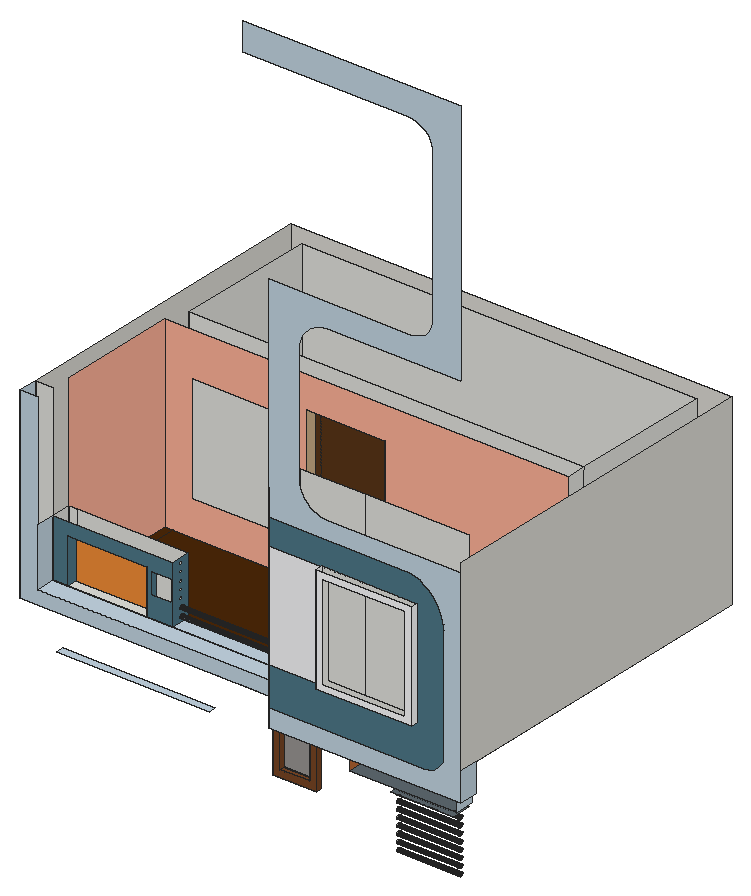
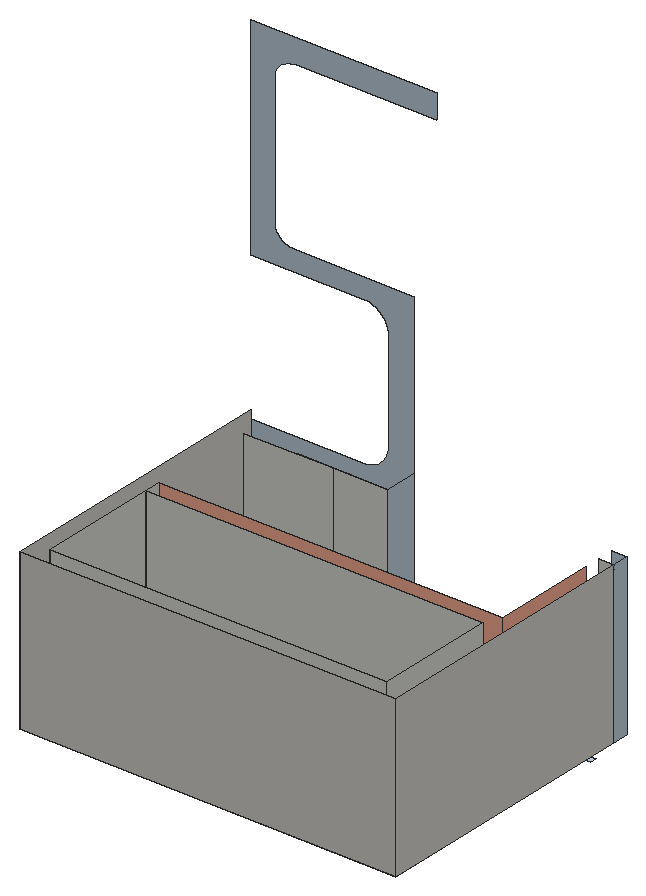
# SketchUp Ruby script. Lengths in inches.
U = 1.inch
M = Sketchup.active_model
def pt(a) = Geom::Point3d.new(a.map { |v| v * U })
def face(e, loops, mat)
  f = e.add_face(loops[0].map { |a| pt(a) })
  loops[1..].each { |l| e.add_face(l.map { |a| pt(a) }).erase! }
  f.material = f.back_material = mat if mat
  f
end
# faces: each face lists its corners as indices into pts; further lists are holes
def faces(e, pts, list, mat = nil) = list.each { |f| face(e, (f[0].is_a?(Array) ? f : [f]).map { |l| l.map { |i| pts[i] } }, mat) }
# xy, xz, yz: faces in a plane at the given z, y or x. An outline is a flat list of corners, or four numbers for a rectangle; further outlines are holes
def ring(l) = l.size == 4 ? [[l[0], l[1]], [l[2], l[1]], [l[2], l[3]], [l[0], l[3]]] : l.each_slice(2).to_a
def flat(e, list, mat, &to3) = list.each { |f| face(e, (f[0].is_a?(Array) ? f : [f]).map { |l| ring(l).map { |u, v| to3.(u, v) } }, mat) }
def xy(e, z, list, mat = nil) = flat(e, list, mat) { |x, y| [x, y, z] }
def xz(e, y, list, mat = nil) = flat(e, list, mat) { |x, z| [x, y, z] }
def yz(e, x, list, mat = nil) = flat(e, list, mat) { |y, z| [x, y, z] }
def lines(e, pts, list) = list.each { |a, b| e.add_line(pt(pts[a]), pt(pts[b])) }
# prism: a flat outline (further loops are holes) pulled along v
def prism(e, loops, v, mat = nil)
  f = face(e, loops, mat); d = Geom::Vector3d.new(v.map { |x| x * U })
  f.pushpull(f.normal.samedirection?(d) ? d.length : -d.length)
end
def box(e, o, s, mat = nil) = prism(e, [[o, [o[0] + s[0], o[1], o[2]], [o[0] + s[0], o[1] + s[1], o[2]], [o[0], o[1] + s[1], o[2]]]], [0, 0, s[2]], mat)
def at(x, y, z, deg = 0) = Geom::Transformation.translation(pt([x, y, z])) * Geom::Transformation.rotation(ORIGIN, Z_AXIS, deg.degrees)
def axes(o, x, y, z) = Geom::Transformation.new([*x, 0, *y, 0, *z, 0, *pt(o).to_a, 1])
def part(name) = M.definitions.add(name)
# library, detail: a bought-in or finely detailed component or shape, given as its bounding box
def library(name, o, s) = part(name).tap { |d| box(d.entities, o, s) }
def detail(e, o, s) = box(e.add_group.entities, o, s)
def put(e, d, t, mat = nil) = e.add_instance(d, t).tap { |i| i.material = mat if mat }
def group(e, t, mat = nil) = e.add_group.tap { |g| g.transformation = t; g.material = mat if mat }.entities
root = M.entities
M.materials.add("[0035_Tan]").color = [210, 180, 140]
M.materials.add("[0096_SkyBlue]").color = [79, 120, 137]
M.materials.add("[Blinds Vertical Pattern]").color = [247, 247, 249]
M.materials.add("[Cladding Siding Tan]").color = [242, 141, 55]
M.materials.add("[Color B02]").color = [255, 178, 153]
M.materials.add("[Concrete Aggregate Smoke]").color = [154, 150, 148]
M.materials.add("[Formica Laminate Dark]").color = [50, 53, 60]
M.materials.add("[Formica Speckled Grey]").color = [94, 105, 111]
M.materials.add("[Leather Red Brown]").color = [76, 40, 8]
M.materials.add("[Quartz Light Grey]").color = [251, 251, 252]
M.materials.add("[Terrazzo Light Blue]").color = [196, 214, 227]
M.materials.add("[Terrazzo Tile Light]").color = [219, 217, 210]
M.materials.add("[Wood Cherry Original]").color = [188, 106, 52]
M.materials.add("[Wood Floor Parquet]").color = [89, 54, 24]
M.materials.add("[Wood Veneer 01]").color = [120, 70, 37]
xy(root,101.78,[[212.44,171.81,240.69,175.06]],"[Wood Veneer 01]")
xy(root,106.21,[[216.87,171.81,236.26,175.06]],"[Wood Veneer 01]")
xy(root,116.03,[[285.76,175.06,326.14,187.5]],"[Formica Speckled Grey]")
xy(root,119,[[259.37,175.06,326.14,187.5],[326.14,175.06,328.05,187.5]],"[Formica Speckled Grey]")
xy(root,129.14,[[79.41,164.37,177.78,169]],"[Terrazzo Light Blue]")
xy(root,129.79,[[216.87,171.81,236.26,175.06]],"[Wood Veneer 01]")
xy(root,134.22,[[212.44,171.81,240.69,175.06]],"[Wood Veneer 01]")
xy(root,134.25,[[217.34,162.87,340.49,175.06]],"[Terrazzo Light Blue]")
xy(root,142.25,[[259.37,175.06,328.05,187.5]])
xy(root,152.8125,[[57.16,162.87,73.72,169],[73.72,162.87,210.68,169],[210.68,162.87,217.34,175.06],[57.16,169,73.72,175.06],[73.72,169,210.68,175.06],
  [73.72,175.06,217.34,187.5],[217.34,175.06,328.05,187.5],[73.72,277.89,328.05,368.29]])
xy(root,152.8125,[[159.93,265.26,209.68,271.64]],"[0035_Tan]")
xy(root,152.8125,[[73.72,265.26,73.72,277.89,328.05,277.89,328.05,265.26,209.68,265.26,209.68,271.64,159.93,271.64,159.93,265.26]],"[Formica Speckled Grey]")
xy(root,152.8125,[[57.16,175.06,57.16,380.73,340.49,380.73,340.49,175.06,328.05,175.06,328.05,368.29,73.72,368.29,73.72,265.26,68.53,265.26,68.53,187.5,73.72,187.5,73.72,175.06],[68.53,187.5,73.72,265.26],[73.72,187.5,328.05,265.26]],"[Leather Red Brown]")
xy(root,161.75,[[68.53,175.06,68.53,187.5,145.53,187.5,145.53,175.06,129.11,175.06,129.11,181.62,77.92,181.62,77.92,175.06],[77.92,175.06,129.11,181.62]])
xy(root,161.75,[[68.53,162.87,217.34,175.06],[145.53,175.06,217.34,187.5]],"[Terrazzo Light Blue]")
xy(root,170.49,[[250.99,158.43,312.37,162.87]],"[Quartz Light Grey]")
xz(root,158.43,[[[250.99,170.49,312.37,239.3],[254.96,174.45,308.4,235.33]]],"[Quartz Light Grey]")
xz(root,162.87,[[[250.99,170.49,312.37,239.3],[254.96,174.45,308.4,235.33]]])
xz(root,162.87,[[217.34,145.51,317.89,145.51,319.24,145.59,320.59,145.84,321.89,146.24,323.15,146.8,324.35,147.51,325.47,148.35,326.49,149.33,327.41,150.42,328.21,151.62,328.89,152.9,329.4375,154.26,329.84,155.67,329.84,227.94,329.62,231.55,328.97,235.1,327.91,238.53,326.4375,241.77,324.6,244.78,322.41,247.5,319.91,249.88,317.15,251.89,314.17,253.49,311.03,254.66,307.78,255.36,304.46,255.6,217.34,255.6,217.34,239.3,312.37,239.3,312.37,170.49,217.34,170.49]],"[0096_SkyBlue]")
xz(root,162.87,[[217.34,170.49,250.99,239.3]],"[Blinds Vertical Pattern]")
xz(root,162.87,[[217.34,134.25,340.49,134.25,340.49,266.71,254.82,266.71,252.4375,266.86,250.1,267.33,247.84,268.09,245.71,269.15,243.72,270.47,241.93,272.04,240.36,273.84,239.04,275.82,237.98,277.95,237.22,280.21,236.75,282.55,236.6,284.93,236.6,358.97,236.75,361.36,237.22,363.71,237.99,365.98,239.05,368.13,240.38,370.125,241.97,371.93,243.77,373.51,245.76,374.84,247.91,375.9,250.18,376.67,252.54,377.14,254.93,377.3,340.49,377.3,340.49,536.0625,200.4,536.0625,200.4,518.04,306.125,518.04,308.3,517.92,310.4375,517.55,312.5,516.9375,314.45,516.1,316.26,515.05,317.9,513.8,319.34,512.375,320.55,510.8,321.51,509.1,322.21,507.31,322.64,505.45,322.78,503.56,322.78,405.53,322.65,403.87,322.28,402.24,321.67,400.66,320.82,399.17,319.76,397.79,318.5,396.54,317.06,395.44,315.47,394.52,313.75,393.78,311.9375,393.25,310.0625,392.92,308.15,392.8125,217.34,392.8125,217.34,255.6,304.46,255.6,307.78,255.36,311.03,254.66,314.17,253.49,317.15,251.89,319.91,249.88,322.41,247.5,324.6,244.78,326.4375,241.77,327.91,238.53,328.97,235.1,329.62,231.55,329.84,227.94,329.84,155.67,329.4375,154.26,328.89,152.9,328.21,151.62,327.41,150.42,326.49,149.33,325.47,148.35,324.35,147.51,323.15,146.8,321.89,146.24,320.59,145.84,319.24,145.59,317.89,145.51,217.34,145.51],[57.16,152.8125,217.34,152.8125,217.34,161.75,68.53,161.75,68.53,272.8125,57.16,272.8125]],"[Terrazzo Light Blue]")
xz(root,171.81,[[[212.44,101.78,240.69,134.22],[216.87,106.21,236.26,129.79]]],"[Wood Veneer 01]")
xz(root,175.06,[[[212.44,101.78,240.69,134.22],[216.87,106.21,236.26,129.79]],[217.34,134.25,259.37,134.25,259.37,142.25,328.05,142.25,328.05,152.8125,217.34,152.8125],[259.37,134.25,328.05,142.25],[328.05,134.25,340.49,142.25],[328.05,142.25,340.49,152.8125],
  [57.16,152.8125,57.16,272.8125,68.53,272.8125,68.53,161.75,217.34,161.75,217.34,152.8125]])
xz(root,175.06,[[[68.53,161.75,77.92,161.75,77.92,190.75,129.11,190.75,129.11,161.75,145.53,161.75,145.53,199,68.53,199],[131.3,175.61,144.73,189.05]]],"[0096_SkyBlue]")
xz(root,175.06,[[216.87,106.21,236.26,129.79]],"[Concrete Aggregate Smoke]")
xz(root,181.62,[[77.92,161.75,129.11,190.75]],"[Cladding Siding Tan]")
xz(root,187.5,[[68.53,152.8125,73.72,161.75],[73.72,152.8125,217.34,161.75],[217.34,152.8125,259.37,272.8125],[259.37,152.8125,326.14,272.8125],[68.53,161.75,73.72,199],
  [73.72,161.75,145.53,199]])
xz(root,265.26,[[[68.53,152.8125,159.93,152.8125,159.93,252.25,209.68,252.25,209.68,152.8125,328.05,152.8125,328.05,272.8125,68.53,272.8125],[85.49,175.17,140.61,244.54]]],"[Color B02]")
xz(root,271.64,[[[159.93,152.8125,209.68,252.25],[163.48,156.36,206.13,248.7]],[163.48,156.36,206.13,248.7]],"[Wood Floor Parquet]")
xz(root,277.89,[[73.72,152.8125,328.05,272.8125]])
xz(root,368.29,[[73.72,152.8125,328.05,272.8125]])
xz(root,380.73,[[57.16,152.8125,340.49,272.8125]],"[Terrazzo Tile Light]")
yz(root,57.16,[[162.87,152.8125,175.06,272.8125]],"[Terrazzo Light Blue]")
yz(root,57.16,[[175.06,152.8125,380.73,272.8125]],"[Terrazzo Tile Light]")
yz(root,68.53,[[175.06,161.75,187.5,199]])
yz(root,68.53,[[187.5,152.8125,265.26,272.8125]],"[Color B02]")
yz(root,68.53,[[162.87,161.75,175.06,199]],"[Terrazzo Light Blue]")
yz(root,73.72,[[277.89,152.8125,368.29,272.8125]])
yz(root,77.92,[[175.06,161.75,181.62,190.75]],"[0096_SkyBlue]")
yz(root,129.11,[[175.06,161.75,181.62,190.75]],"[0096_SkyBlue]")
yz(root,145.53,[[181.52,164.09,181.21,164.125,180.92,164.24,180.68,164.43,180.49,164.68,180.37,164.97,180.33,165.27,180.37,165.58,180.49,165.87,180.68,166.11,180.92,166.3,181.21,166.42,181.52,166.46,181.82,166.42,182.11,166.3,182.35,166.11,182.54,165.87,182.66,165.58,182.7,165.27,182.66,164.97,182.54,164.68,182.35,164.43,182.11,164.24,181.82,164.125],[181.52,169.34,181.21,169.375,180.92,169.49,180.68,169.68,180.49,169.93,180.37,170.22,180.33,170.52,180.37,170.83,180.49,171.12,180.68,171.36,180.92,171.55,181.21,171.67,181.52,171.71,181.82,171.67,182.11,171.55,182.35,171.36,182.54,171.12,182.66,170.83,182.7,170.52,182.66,170.22,182.54,169.93,182.35,169.68,182.11,169.49,181.82,169.375]])
yz(root,145.53,[[[175.06,161.75,187.5,199],[181.52,164.09,181.21,164.125,180.92,164.24,180.68,164.43,180.49,164.68,180.37,164.97,180.33,165.27,180.37,165.58,180.49,165.87,180.68,166.11,180.92,166.3,181.21,166.42,181.52,166.46,181.82,166.42,182.11,166.3,182.35,166.11,182.54,165.87,182.66,165.58,182.7,165.27,182.66,164.97,182.54,164.68,182.35,164.43,182.11,164.24,181.82,164.125],[181.52,189.77,181.21,189.8125,180.92,189.93,180.68,190.12,180.49,190.37,180.37,190.65,180.33,190.96,180.37,191.27,180.49,191.55,180.68,191.8,180.92,191.99,181.21,192.11,181.52,192.15,181.82,192.11,182.11,191.99,182.35,191.8,182.54,191.55,182.66,191.27,182.7,190.96,182.66,190.65,182.54,190.37,182.35,190.12,182.11,189.93,181.82,189.8125],[181.52,169.34,181.21,169.375,180.92,169.49,180.68,169.68,180.49,169.93,180.37,170.22,180.33,170.52,180.37,170.83,180.49,171.12,180.68,171.36,180.92,171.55,181.21,171.67,181.52,171.71,181.82,171.67,182.11,171.55,182.35,171.36,182.54,171.12,182.66,170.83,182.7,170.52,182.66,170.22,182.54,169.93,182.35,169.68,182.11,169.49,181.82,169.375],[181.52,184.52,181.21,184.5625,180.92,184.68,180.68,184.87,180.49,185.12,180.37,185.4,180.33,185.71,180.37,186.02,180.49,186.3,180.68,186.55,180.92,186.74,181.21,186.86,181.52,186.9,181.82,186.86,182.11,186.74,182.35,186.55,182.54,186.3,182.66,186.02,182.7,185.71,182.66,185.4,182.54,185.12,182.35,184.87,182.11,184.68,181.82,184.5625],[181.52,174.46,181.21,174.5,180.92,174.62,180.68,174.81,180.49,175.05,180.37,175.34,180.33,175.65,180.37,175.96,180.49,176.24,180.68,176.49,180.92,176.68,181.21,176.8,181.52,176.84,181.82,176.8,182.11,176.68,182.35,176.49,182.54,176.24,182.66,175.96,182.7,175.65,182.66,175.34,182.54,175.05,182.35,174.81,182.11,174.62,181.82,174.5],[181.52,179.59,181.21,179.625,180.92,179.74,180.68,179.93,180.49,180.18,180.37,180.47,180.33,180.77,180.37,181.08,180.49,181.37,180.68,181.61,180.92,181.8,181.21,181.92,181.52,181.96,181.82,181.92,182.11,181.8,182.35,181.61,182.54,181.37,182.66,181.08,182.7,180.77,182.66,180.47,182.54,180.18,182.35,179.93,182.11,179.74,181.82,179.625],[181.52,194.9,181.21,194.9375,180.92,195.06,180.68,195.25,180.49,195.49,180.37,195.78,180.33,196.09,180.37,196.39,180.49,196.68,180.68,196.93,180.92,197.11,181.21,197.23,181.52,197.27,181.82,197.23,182.11,197.11,182.35,196.93,182.54,196.68,182.66,196.39,182.7,196.09,182.66,195.78,182.54,195.49,182.35,195.25,182.11,195.06,181.82,194.9375]]],"[0096_SkyBlue]")
yz(root,159.93,[[265.26,152.8125,271.64,252.25]],"[0035_Tan]")
yz(root,209.68,[[265.26,152.8125,271.64,252.25]],"[0035_Tan]")
yz(root,212.44,[[171.81,101.78,175.06,134.22]],"[Wood Veneer 01]")
yz(root,216.87,[[171.81,106.21,175.06,129.79]],"[Wood Veneer 01]")
yz(root,217.34,[[162.87,134.25,175.06,152.8125],[162.87,152.8125,175.06,161.75],[175.06,152.8125,187.5,161.75]])
yz(root,217.34,[[[162.87,161.75,187.5,272.8125],[181.52,194.9,181.82,194.9375,182.11,195.06,182.35,195.25,182.54,195.49,182.66,195.78,182.7,196.09,182.66,196.39,182.54,196.68,182.35,196.93,182.11,197.11,181.82,197.23,181.52,197.27,181.21,197.23,180.92,197.11,180.68,196.93,180.49,196.68,180.37,196.39,180.33,196.09,180.37,195.78,180.49,195.49,180.68,195.25,180.92,195.06,181.21,194.9375],[181.52,164.09,181.82,164.125,182.11,164.24,182.35,164.43,182.54,164.68,182.66,164.97,182.7,165.27,182.66,165.58,182.54,165.87,182.35,166.11,182.11,166.3,181.82,166.42,181.52,166.46,181.21,166.42,180.92,166.3,180.68,166.11,180.49,165.87,180.37,165.58,180.33,165.27,180.37,164.97,180.49,164.68,180.68,164.43,180.92,164.24,181.21,164.125],[181.52,169.34,181.82,169.375,182.11,169.49,182.35,169.68,182.54,169.93,182.66,170.22,182.7,170.52,182.66,170.83,182.54,171.12,182.35,171.36,182.11,171.55,181.82,171.67,181.52,171.71,181.21,171.67,180.92,171.55,180.68,171.36,180.49,171.12,180.37,170.83,180.33,170.52,180.37,170.22,180.49,169.93,180.68,169.68,180.92,169.49,181.21,169.375],[181.52,174.46,181.82,174.5,182.11,174.62,182.35,174.81,182.54,175.05,182.66,175.34,182.7,175.65,182.66,175.96,182.54,176.24,182.35,176.49,182.11,176.68,181.82,176.8,181.52,176.84,181.21,176.8,180.92,176.68,180.68,176.49,180.49,176.24,180.37,175.96,180.33,175.65,180.37,175.34,180.49,175.05,180.68,174.81,180.92,174.62,181.21,174.5],[181.52,179.59,181.82,179.625,182.11,179.74,182.35,179.93,182.54,180.18,182.66,180.47,182.7,180.77,182.66,181.08,182.54,181.37,182.35,181.61,182.11,181.8,181.82,181.92,181.52,181.96,181.21,181.92,180.92,181.8,180.68,181.61,180.49,181.37,180.37,181.08,180.33,180.77,180.37,180.47,180.49,180.18,180.68,179.93,180.92,179.74,181.21,179.625],[181.52,184.52,181.82,184.5625,182.11,184.68,182.35,184.87,182.54,185.12,182.66,185.4,182.7,185.71,182.66,186.02,182.54,186.3,182.35,186.55,182.11,186.74,181.82,186.86,181.52,186.9,181.21,186.86,180.92,186.74,180.68,186.55,180.49,186.3,180.37,186.02,180.33,185.71,180.37,185.4,180.49,185.12,180.68,184.87,180.92,184.68,181.21,184.5625],[181.52,189.77,181.82,189.8125,182.11,189.93,182.35,190.12,182.54,190.37,182.66,190.65,182.7,190.96,182.66,191.27,182.54,191.55,182.35,191.8,182.11,191.99,181.82,192.11,181.52,192.15,181.21,192.11,180.92,191.99,180.68,191.8,180.49,191.55,180.37,191.27,180.33,190.96,180.37,190.65,180.49,190.37,180.68,190.12,180.92,189.93,181.21,189.8125]]],"[Terrazzo Light Blue]")
yz(root,236.26,[[171.81,106.21,175.06,129.79]],"[Wood Veneer 01]")
yz(root,240.69,[[171.81,101.78,175.06,134.22]],"[Wood Veneer 01]")
yz(root,250.99,[[158.43,170.49,162.87,239.3]],"[Quartz Light Grey]")
yz(root,259.37,[[175.06,119,187.5,142.25]],"[Wood Cherry Original]")
yz(root,285.76,[[181.25,78.9,180.96,78.94,180.6875,79.05,180.45,79.23,180.28,79.47,180.16,79.74,180.125,80.03,180.16,80.32,180.28,80.59,180.45,80.82,180.6875,81,180.96,81.12,181.25,81.15,181.54,81.12,181.8125,81,182.05,80.82,182.22,80.59,182.34,80.32,182.375,80.03,182.34,79.74,182.22,79.47,182.05,79.23,181.8125,79.05,181.54,78.94],[181.25,83.59,180.96,83.63,180.6875,83.74,180.45,83.92,180.28,84.15,180.16,84.42,180.125,84.72,180.16,85.01,180.28,85.28,180.45,85.51,180.6875,85.69,180.96,85.8,181.25,85.84,181.54,85.8,181.8125,85.69,182.05,85.51,182.22,85.28,182.34,85.01,182.375,84.72,182.34,84.42,182.22,84.15,182.05,83.92,181.8125,83.74,181.54,83.63],[181.25,88.28,180.96,88.32,180.6875,88.43,180.45,88.61,180.28,88.84,180.16,89.11,180.125,89.4,180.16,89.69,180.28,89.97,180.45,90.2,180.6875,90.38,180.96,90.49,181.25,90.53,181.54,90.49,181.8125,90.38,182.05,90.2,182.22,89.97,182.34,89.69,182.375,89.4,182.34,89.11,182.22,88.84,182.05,88.61,181.8125,88.43,181.54,88.32],[181.25,92.97,180.96,93,180.6875,93.12,180.45,93.3,180.28,93.53,180.16,93.8,180.125,94.09,180.16,94.38,180.28,94.65,180.45,94.89,180.6875,95.07,180.96,95.18,181.25,95.22,181.54,95.18,181.8125,95.07,182.05,94.89,182.22,94.65,182.34,94.38,182.375,94.09,182.34,93.8,182.22,93.53,182.05,93.3,181.8125,93.12,181.54,93],[181.25,97.65,180.96,97.69,180.6875,97.8,180.45,97.98,180.28,98.22,180.16,98.49,180.125,98.78,180.16,99.07,180.28,99.34,180.45,99.57,180.6875,99.75,180.96,99.87,181.25,99.9,181.54,99.87,181.8125,99.75,182.05,99.57,182.22,99.34,182.34,99.07,182.375,98.78,182.34,98.49,182.22,98.22,182.05,97.98,181.8125,97.8,181.54,97.69],
  [181.25,102.34,180.96,102.38,180.6875,102.49,180.45,102.67,180.28,102.9,180.16,103.17,180.125,103.47,180.16,103.76,180.28,104.03,180.45,104.26,180.6875,104.44,180.96,104.55,181.25,104.59,181.54,104.55,181.8125,104.44,182.05,104.26,182.22,104.03,182.34,103.76,182.375,103.47,182.34,103.17,182.22,102.9,182.05,102.67,181.8125,102.49,181.54,102.38],[181.25,107.03,180.96,107.07,180.6875,107.18,180.45,107.36,180.28,107.59,180.16,107.86,180.125,108.15,180.16,108.44,180.28,108.72,180.45,108.95,180.6875,109.13,180.96,109.24,181.25,109.28,181.54,109.24,181.8125,109.13,182.05,108.95,182.22,108.72,182.34,108.44,182.375,108.15,182.34,107.86,182.22,107.59,182.05,107.36,181.8125,107.18,181.54,107.07],[181.25,111.72,180.96,111.75,180.6875,111.87,180.45,112.05,180.28,112.28,180.16,112.55,180.125,112.84,180.16,113.13,180.28,113.4,180.45,113.64,180.6875,113.82,180.96,113.93,181.25,113.97,181.54,113.93,181.8125,113.82,182.05,113.64,182.22,113.4,182.34,113.13,182.375,112.84,182.34,112.55,182.22,112.28,182.05,112.05,181.8125,111.87,181.54,111.75]])
yz(root,312.37,[[158.43,170.49,162.87,239.3]],"[Quartz Light Grey]")
yz(root,328.05,[[175.06,142.25,187.5,152.8125],[265.26,152.8125,277.89,272.8125],[277.89,152.8125,368.29,272.8125]])
yz(root,328.05,[[175.06,119,187.5,142.25]],"[Terrazzo Light Blue]")
yz(root,340.49,[[162.87,134.25,175.06,152.8125]],"[Terrazzo Light Blue]")
yz(root,340.49,[[162.87,152.8125,380.73,272.8125]],"[Terrazzo Tile Light]")
p = [[285.76,180.6875,79.05],[285.76,180.96,78.94],[326.14,180.96,78.94],[326.14,180.6875,79.05],[285.76,181.25,78.9],[326.14,181.25,78.9],
  [285.76,181.54,78.94],[326.14,181.54,78.94],[285.76,181.8125,79.05],[326.14,181.8125,79.05],[285.76,180.45,79.23],[326.14,180.45,79.23],
  [285.76,182.05,79.23],[326.14,182.05,79.23],[285.76,180.28,79.47],[326.14,180.28,79.47],[285.76,182.22,79.47],[326.14,182.22,79.47],
  [285.76,180.16,79.74],[326.14,180.16,79.74],[285.76,182.34,79.74],[326.14,182.34,79.74],[285.76,180.125,80.03],[326.14,180.125,80.03],
  [285.76,182.375,80.03],[326.14,182.375,80.03],[285.76,180.16,80.32],[326.14,180.16,80.32],[285.76,182.34,80.32],[326.14,182.34,80.32],
  [285.76,180.28,80.59],[326.14,180.28,80.59],[285.76,182.22,80.59],[326.14,182.22,80.59],[285.76,180.45,80.82],[326.14,180.45,80.82],
  [285.76,182.05,80.82],[326.14,182.05,80.82],[285.76,180.6875,81],[326.14,180.6875,81],[285.76,181.8125,81],[326.14,181.8125,81],
  [285.76,180.96,81.12],[326.14,180.96,81.12],[285.76,181.54,81.12],[326.14,181.54,81.12],[285.76,181.25,81.15],[326.14,181.25,81.15],
  [285.76,180.6875,83.74],[285.76,180.96,83.63],[326.14,180.96,83.63],[326.14,180.6875,83.74],[285.76,181.25,83.59],[326.14,181.25,83.59],
  [285.76,181.54,83.63],[326.14,181.54,83.63],[285.76,181.8125,83.74],[326.14,181.8125,83.74],[285.76,180.45,83.92],[326.14,180.45,83.92],
  [285.76,182.05,83.92],[326.14,182.05,83.92],[285.76,180.28,84.15],[326.14,180.28,84.15],[285.76,182.22,84.15],[326.14,182.22,84.15],
  [285.76,180.16,84.42],[326.14,180.16,84.42],[285.76,182.34,84.42],[326.14,182.34,84.42],[285.76,180.125,84.72],[326.14,180.125,84.72],
  [285.76,182.375,84.72],[326.14,182.375,84.72],[285.76,180.16,85.01],[326.14,180.16,85.01],[285.76,182.34,85.01],[326.14,182.34,85.01],
  [285.76,180.28,85.28],[326.14,180.28,85.28],[285.76,182.22,85.28],[326.14,182.22,85.28],[285.76,180.45,85.51],[326.14,180.45,85.51],
  [285.76,182.05,85.51],[326.14,182.05,85.51],[285.76,180.6875,85.69],[326.14,180.6875,85.69],[285.76,181.8125,85.69],[326.14,181.8125,85.69],
  [285.76,180.96,85.8],[326.14,180.96,85.8],[285.76,181.54,85.8],[326.14,181.54,85.8],[285.76,181.25,85.84],[326.14,181.25,85.84],
  [285.76,180.6875,88.43],[285.76,180.96,88.32],[326.14,180.96,88.32],[326.14,180.6875,88.43],[285.76,181.25,88.28],[326.14,181.25,88.28],
  [285.76,181.54,88.32],[326.14,181.54,88.32],[285.76,181.8125,88.43],[326.14,181.8125,88.43],[285.76,180.45,88.61],[326.14,180.45,88.61],
  [285.76,182.05,88.61],[326.14,182.05,88.61],[285.76,180.28,88.84],[326.14,180.28,88.84],[285.76,182.22,88.84],[326.14,182.22,88.84],
  [285.76,180.16,89.11],[326.14,180.16,89.11],[285.76,182.34,89.11],[326.14,182.34,89.11],[285.76,180.125,89.4],[326.14,180.125,89.4],
  [285.76,182.375,89.4],[326.14,182.375,89.4],[285.76,180.16,89.69],[326.14,180.16,89.69],[285.76,182.34,89.69],[326.14,182.34,89.69],
  [285.76,180.28,89.97],[326.14,180.28,89.97],[285.76,182.22,89.97],[326.14,182.22,89.97],[285.76,180.45,90.2],[326.14,180.45,90.2],
  [285.76,182.05,90.2],[326.14,182.05,90.2],[285.76,180.6875,90.38],[326.14,180.6875,90.38],[285.76,181.8125,90.38],[326.14,181.8125,90.38],
  [285.76,180.96,90.49],[326.14,180.96,90.49],[285.76,181.54,90.49],[326.14,181.54,90.49],[285.76,181.25,90.53],[326.14,181.25,90.53],
  [285.76,180.6875,93.12],[285.76,180.96,93],[326.14,180.96,93],[326.14,180.6875,93.12],[285.76,181.25,92.97],[326.14,181.25,92.97],
  [285.76,181.54,93],[326.14,181.54,93],[285.76,181.8125,93.12],[326.14,181.8125,93.12],[285.76,180.45,93.3],[326.14,180.45,93.3],
  [285.76,182.05,93.3],[326.14,182.05,93.3],[285.76,180.28,93.53],[326.14,180.28,93.53],[285.76,182.22,93.53],[326.14,182.22,93.53],
  [285.76,180.16,93.8],[326.14,180.16,93.8],[285.76,182.34,93.8],[326.14,182.34,93.8],[285.76,180.125,94.09],[326.14,180.125,94.09],
  [285.76,182.375,94.09],[326.14,182.375,94.09],[285.76,180.16,94.38],[326.14,180.16,94.38],[285.76,182.34,94.38],[326.14,182.34,94.38],
  [285.76,180.28,94.65],[326.14,180.28,94.65],[285.76,182.22,94.65],[326.14,182.22,94.65],[285.76,180.45,94.89],[326.14,180.45,94.89],
  [285.76,182.05,94.89],[326.14,182.05,94.89],[285.76,180.6875,95.07],[326.14,180.6875,95.07],[285.76,181.8125,95.07],[326.14,181.8125,95.07],
  [285.76,180.96,95.18],[326.14,180.96,95.18],[285.76,181.54,95.18],[326.14,181.54,95.18],[285.76,181.25,95.22],[326.14,181.25,95.22],
  [285.76,180.6875,97.8],[285.76,180.96,97.69],[326.14,180.96,97.69],[326.14,180.6875,97.8],[285.76,181.25,97.65],[326.14,181.25,97.65],
  [285.76,181.54,97.69],[326.14,181.54,97.69],[285.76,181.8125,97.8],[326.14,181.8125,97.8],[285.76,180.45,97.98],[326.14,180.45,97.98],
  [285.76,182.05,97.98],[326.14,182.05,97.98],[285.76,180.28,98.22],[326.14,180.28,98.22],[285.76,182.22,98.22],[326.14,182.22,98.22],
  [285.76,180.16,98.49],[326.14,180.16,98.49],[285.76,182.34,98.49],[326.14,182.34,98.49],[285.76,180.125,98.78],[326.14,180.125,98.78],
  [285.76,182.375,98.78],[326.14,182.375,98.78],[285.76,180.16,99.07],[326.14,180.16,99.07],[285.76,182.34,99.07],[326.14,182.34,99.07],
  [285.76,180.28,99.34],[326.14,180.28,99.34],[285.76,182.22,99.34],[326.14,182.22,99.34],[285.76,180.45,99.57],[326.14,180.45,99.57],
  [285.76,182.05,99.57],[326.14,182.05,99.57],[285.76,180.6875,99.75],[326.14,180.6875,99.75],[285.76,181.8125,99.75],[326.14,181.8125,99.75],
  [285.76,180.96,99.87],[326.14,180.96,99.87],[285.76,181.54,99.87],[326.14,181.54,99.87],[285.76,181.25,99.9],[326.14,181.25,99.9],
  [285.76,180.96,102.38],[285.76,181.25,102.34],[326.14,181.25,102.34],[326.14,180.96,102.38],[285.76,181.54,102.38],[326.14,181.54,102.38],
  [285.76,180.6875,102.49],[326.14,180.6875,102.49],[285.76,181.8125,102.49],[326.14,181.8125,102.49],[285.76,180.45,102.67],[326.14,180.45,102.67],
  [285.76,182.05,102.67],[326.14,182.05,102.67],[285.76,180.28,102.9],[326.14,180.28,102.9],[285.76,182.22,102.9],[326.14,182.22,102.9],
  [285.76,180.16,103.17],[326.14,180.16,103.17],[285.76,182.34,103.17],[326.14,182.34,103.17],[285.76,180.125,103.47],[326.14,180.125,103.47],
  [285.76,182.375,103.47],[326.14,182.375,103.47],[285.76,180.16,103.76],[326.14,180.16,103.76],[285.76,182.34,103.76],[326.14,182.34,103.76],
  [285.76,180.28,104.03],[326.14,180.28,104.03],[285.76,182.22,104.03],[326.14,182.22,104.03],[285.76,180.45,104.26],[326.14,180.45,104.26],
  [285.76,182.05,104.26],[326.14,182.05,104.26],[285.76,180.6875,104.44],[326.14,180.6875,104.44],[285.76,181.8125,104.44],[326.14,181.8125,104.44],
  [285.76,180.96,104.55],[326.14,180.96,104.55],[285.76,181.54,104.55],[326.14,181.54,104.55],[285.76,181.25,104.59],[326.14,181.25,104.59],
  [285.76,180.96,107.07],[285.76,181.25,107.03],[326.14,181.25,107.03],[326.14,180.96,107.07],[285.76,181.54,107.07],[326.14,181.54,107.07],
  [285.76,180.6875,107.18],[326.14,180.6875,107.18],[285.76,181.8125,107.18],[326.14,181.8125,107.18],[285.76,180.45,107.36],[326.14,180.45,107.36],
  [285.76,182.05,107.36],[326.14,182.05,107.36],[285.76,180.28,107.59],[326.14,180.28,107.59],[285.76,182.22,107.59],[326.14,182.22,107.59],
  [285.76,180.16,107.86],[326.14,180.16,107.86],[285.76,182.34,107.86],[326.14,182.34,107.86],[285.76,180.125,108.15],[326.14,180.125,108.15],
  [285.76,182.375,108.15],[326.14,182.375,108.15],[285.76,180.16,108.44],[326.14,180.16,108.44],[285.76,182.34,108.44],[326.14,182.34,108.44],
  [285.76,180.28,108.72],[326.14,180.28,108.72],[285.76,182.22,108.72],[326.14,182.22,108.72],[285.76,180.45,108.95],[326.14,180.45,108.95],
  [285.76,182.05,108.95],[326.14,182.05,108.95],[285.76,180.6875,109.13],[326.14,180.6875,109.13],[285.76,181.8125,109.13],[326.14,181.8125,109.13],
  [285.76,180.96,109.24],[326.14,180.96,109.24],[285.76,181.54,109.24],[326.14,181.54,109.24],[285.76,181.25,109.28],[326.14,181.25,109.28],
  [285.76,180.96,111.75],[285.76,181.25,111.72],[326.14,181.25,111.72],[326.14,180.96,111.75],[285.76,181.54,111.75],[326.14,181.54,111.75],
  [285.76,180.6875,111.87],[326.14,180.6875,111.87],[285.76,181.8125,111.87],[326.14,181.8125,111.87],[285.76,180.45,112.05],[326.14,180.45,112.05],
  [285.76,182.05,112.05],[326.14,182.05,112.05],[285.76,180.28,112.28],[326.14,180.28,112.28],[285.76,182.22,112.28],[326.14,182.22,112.28],
  [285.76,180.16,112.55],[326.14,180.16,112.55],[285.76,182.34,112.55],[326.14,182.34,112.55],[285.76,180.125,112.84],[326.14,180.125,112.84],
  [285.76,182.375,112.84],[326.14,182.375,112.84],[285.76,180.16,113.13],[326.14,180.16,113.13],[285.76,182.34,113.13],[326.14,182.34,113.13],
  [285.76,180.28,113.4],[326.14,180.28,113.4],[285.76,182.22,113.4],[326.14,182.22,113.4],[285.76,180.45,113.64],[326.14,180.45,113.64],
  [285.76,182.05,113.64],[326.14,182.05,113.64],[285.76,180.6875,113.82],[326.14,180.6875,113.82],[285.76,181.8125,113.82],[326.14,181.8125,113.82],
  [285.76,180.96,113.93],[326.14,180.96,113.93],[285.76,181.54,113.93],[326.14,181.54,113.93],[285.76,181.25,113.97],[326.14,181.25,113.97],
  [145.53,180.92,164.24],[145.53,181.21,164.125],[217.34,181.21,164.125],[217.34,180.92,164.24],[145.53,181.52,164.09],[217.34,181.52,164.09],
  [145.53,181.82,164.125],[217.34,181.82,164.125],[145.53,182.11,164.24],[217.34,182.11,164.24],[145.53,180.68,164.43],[217.34,180.68,164.43],
  [145.53,182.35,164.43],[217.34,182.35,164.43],[145.53,180.49,164.68],[217.34,180.49,164.68],[145.53,182.54,164.68],[217.34,182.54,164.68],
  [145.53,180.37,164.97],[217.34,180.37,164.97],[145.53,182.66,164.97],[217.34,182.66,164.97],[145.53,180.33,165.27],[217.34,180.33,165.27],
  [145.53,182.7,165.27],[217.34,182.7,165.27],[145.53,180.37,165.58],[217.34,180.37,165.58],[145.53,182.66,165.58],[217.34,182.66,165.58],
  [145.53,180.49,165.87],[217.34,180.49,165.87],[145.53,182.54,165.87],[217.34,182.54,165.87],[145.53,180.68,166.11],[217.34,180.68,166.11],
  [145.53,182.35,166.11],[217.34,182.35,166.11],[145.53,180.92,166.3],[217.34,180.92,166.3],[145.53,182.11,166.3],[217.34,182.11,166.3],
  [145.53,181.21,166.42],[217.34,181.21,166.42],[145.53,181.82,166.42],[217.34,181.82,166.42],[145.53,181.52,166.46],[217.34,181.52,166.46],
  [145.53,181.21,169.375],[145.53,181.52,169.34],[217.34,181.52,169.34],[217.34,181.21,169.375],[145.53,181.82,169.375],[217.34,181.82,169.375],
  [145.53,180.92,169.49],[217.34,180.92,169.49],[145.53,182.11,169.49],[217.34,182.11,169.49],[145.53,180.68,169.68],[217.34,180.68,169.68],
  [145.53,182.35,169.68],[217.34,182.35,169.68],[145.53,180.49,169.93],[217.34,180.49,169.93],[145.53,182.54,169.93],[217.34,182.54,169.93],
  [145.53,180.37,170.22],[217.34,180.37,170.22],[145.53,182.66,170.22],[217.34,182.66,170.22],[145.53,180.33,170.52],[217.34,180.33,170.52],
  [145.53,182.7,170.52],[217.34,182.7,170.52],[145.53,180.37,170.83],[217.34,180.37,170.83],[145.53,182.66,170.83],[217.34,182.66,170.83],
  [145.53,180.49,171.12],[217.34,180.49,171.12],[145.53,182.54,171.12],[217.34,182.54,171.12],[145.53,180.68,171.36],[217.34,180.68,171.36],
  [145.53,182.35,171.36],[217.34,182.35,171.36],[145.53,180.92,171.55],[217.34,180.92,171.55],[145.53,182.11,171.55],[217.34,182.11,171.55],
  [145.53,181.21,171.67],[217.34,181.21,171.67],[145.53,181.82,171.67],[217.34,181.82,171.67],[145.53,181.52,171.71],[217.34,181.52,171.71],
  [328.05,175.06,152.8125],[328.05,162.87,152.8125]]
faces(root,p,[[0,1,2,3],[1,4,5,2],[4,6,7,5],[6,8,9,7],[10,0,3,11],[8,12,13,9],[14,10,11,15],[12,16,17,13],
  [18,14,15,19],[16,20,21,17],[22,18,19,23],[20,24,25,21],[26,22,23,27],[24,28,29,25],[30,26,27,31],[28,32,33,29],
  [34,30,31,35],[32,36,37,33],[38,34,35,39],[36,40,41,37],[42,38,39,43],[40,44,45,41],[46,42,43,47],[44,46,47,45],
  [48,49,50,51],[49,52,53,50],[52,54,55,53],[54,56,57,55],[58,48,51,59],[56,60,61,57],[62,58,59,63],[60,64,65,61],
  [66,62,63,67],[64,68,69,65],[70,66,67,71],[68,72,73,69],[74,70,71,75],[72,76,77,73],[78,74,75,79],[76,80,81,77],
  [82,78,79,83],[80,84,85,81],[86,82,83,87],[84,88,89,85],[90,86,87,91],[88,92,93,89],[94,90,91,95],[92,94,95,93],
  [96,97,98,99],[97,100,101,98],[100,102,103,101],[102,104,105,103],[106,96,99,107],[104,108,109,105],[110,106,107,111],[108,112,113,109],
  [114,110,111,115],[112,116,117,113],[118,114,115,119],[116,120,121,117],[122,118,119,123],[120,124,125,121],[126,122,123,127],[124,128,129,125],
  [130,126,127,131],[128,132,133,129],[134,130,131,135],[132,136,137,133],[138,134,135,139],[136,140,141,137],[142,138,139,143],[140,142,143,141],
  [144,145,146,147],[145,148,149,146],[148,150,151,149],[150,152,153,151],[154,144,147,155],[152,156,157,153],[158,154,155,159],[156,160,161,157],
  [162,158,159,163],[160,164,165,161],[166,162,163,167],[164,168,169,165],[170,166,167,171],[168,172,173,169],[174,170,171,175],[172,176,177,173],
  [178,174,175,179],[176,180,181,177],[182,178,179,183],[180,184,185,181],[186,182,183,187],[184,188,189,185],[190,186,187,191],[188,190,191,189],
  [192,193,194,195],[193,196,197,194],[196,198,199,197],[198,200,201,199],[202,192,195,203],[200,204,205,201],[206,202,203,207],[204,208,209,205],
  [210,206,207,211],[208,212,213,209],[214,210,211,215],[212,216,217,213],[218,214,215,219],[216,220,221,217],[222,218,219,223],[220,224,225,221],
  [226,222,223,227],[224,228,229,225],[230,226,227,231],[228,232,233,229],[234,230,231,235],[232,236,237,233],[238,234,235,239],[236,238,239,237],
  [240,241,242,243],[241,244,245,242],[246,240,243,247],[244,248,249,245],[250,246,247,251],[248,252,253,249],[254,250,251,255],[252,256,257,253],
  [258,254,255,259],[256,260,261,257],[262,258,259,263],[260,264,265,261],[266,262,263,267],[264,268,269,265],[270,266,267,271],[268,272,273,269],
  [274,270,271,275],[272,276,277,273],[278,274,275,279],[276,280,281,277],[282,278,279,283],[280,284,285,281],[286,282,283,287],[284,286,287,285],
  [288,289,290,291],[289,292,293,290],[294,288,291,295],[292,296,297,293],[298,294,295,299],[296,300,301,297],[302,298,299,303],[300,304,305,301],
  [306,302,303,307],[304,308,309,305],[310,306,307,311],[308,312,313,309],[314,310,311,315],[312,316,317,313],[318,314,315,319],[316,320,321,317],
  [322,318,319,323],[320,324,325,321],[326,322,323,327],[324,328,329,325],[330,326,327,331],[328,332,333,329],[334,330,331,335],[332,334,335,333],
  [336,337,338,339],[337,340,341,338],[342,336,339,343],[340,344,345,341],[346,342,343,347],[344,348,349,345],[350,346,347,351],[348,352,353,349],
  [354,350,351,355],[352,356,357,353],[358,354,355,359],[356,360,361,357],[362,358,359,363],[360,364,365,361],[366,362,363,367],[364,368,369,365],
  [370,366,367,371],[368,372,373,369],[374,370,371,375],[372,376,377,373],[378,374,375,379],[376,380,381,377],[382,378,379,383],[380,382,383,381]],"[Formica Laminate Dark]")
faces(root,p,[[384,385,386,387],[385,388,389,386],[388,390,391,389],[390,392,393,391],[394,384,387,395],[392,396,397,393],[398,394,395,399],[396,400,401,397],
  [402,398,399,403],[400,404,405,401],[406,402,403,407],[404,408,409,405],[410,406,407,411],[408,412,413,409],[414,410,411,415],[412,416,417,413],
  [418,414,415,419],[416,420,421,417],[422,418,419,423],[420,424,425,421],[426,422,423,427],[424,428,429,425],[430,426,427,431],[428,430,431,429],
  [432,433,434,435],[433,436,437,434],[438,432,435,439],[436,440,441,437],[442,438,439,443],[440,444,445,441],[446,442,443,447],[444,448,449,445],
  [450,446,447,451],[448,452,453,449],[454,450,451,455],[452,456,457,453],[458,454,455,459],[456,460,461,457],[462,458,459,463],[460,464,465,461],
  [466,462,463,467],[464,468,469,465],[470,466,467,471],[468,472,473,469],[474,470,471,475],[472,476,477,473],[478,474,475,479],[476,478,479,477]],"[Formica Speckled Grey]")
lines(root,p,[[480,481]])
